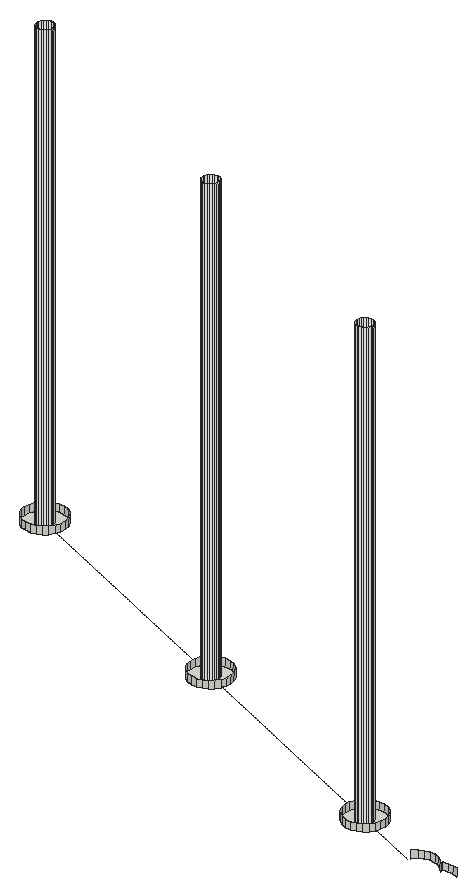
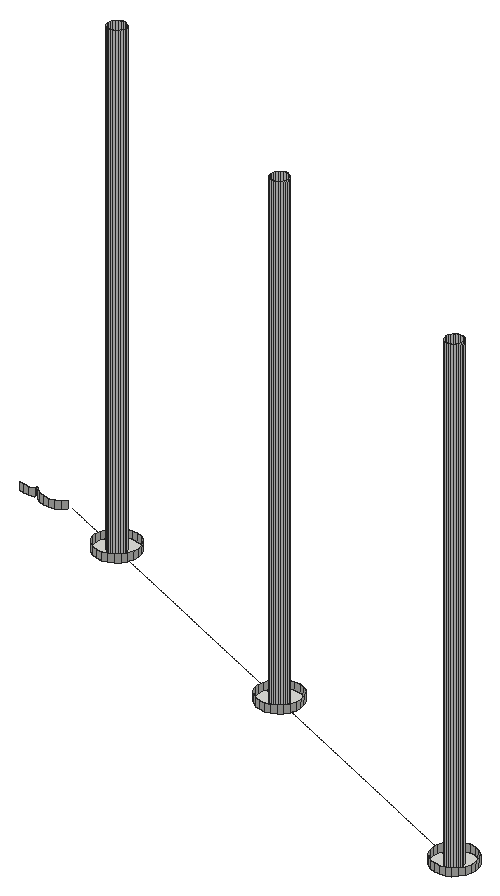
# SketchUp Ruby script. Lengths in inches.
U = 1.inch
M = Sketchup.active_model
def pt(a) = Geom::Point3d.new(a.map { |v| v * U })
def face(e, loops, mat)
  f = e.add_face(loops[0].map { |a| pt(a) })
  loops[1..].each { |l| e.add_face(l.map { |a| pt(a) }).erase! }
  f.material = f.back_material = mat if mat
  f
end
# faces: each face lists its corners as indices into pts; further lists are holes
def faces(e, pts, list, mat = nil) = list.each { |f| face(e, (f[0].is_a?(Array) ? f : [f]).map { |l| l.map { |i| pts[i] } }, mat) }
# xy, xz, yz: faces in a plane at the given z, y or x. An outline is a flat list of corners, or four numbers for a rectangle; further outlines are holes
def ring(l) = l.size == 4 ? [[l[0], l[1]], [l[2], l[1]], [l[2], l[3]], [l[0], l[3]]] : l.each_slice(2).to_a
def flat(e, list, mat, &to3) = list.each { |f| face(e, (f[0].is_a?(Array) ? f : [f]).map { |l| ring(l).map { |u, v| to3.(u, v) } }, mat) }
def xy(e, z, list, mat = nil) = flat(e, list, mat) { |x, y| [x, y, z] }
def xz(e, y, list, mat = nil) = flat(e, list, mat) { |x, z| [x, y, z] }
def yz(e, x, list, mat = nil) = flat(e, list, mat) { |y, z| [x, y, z] }
def lines(e, pts, list) = list.each { |a, b| e.add_line(pt(pts[a]), pt(pts[b])) }
# prism: a flat outline (further loops are holes) pulled along v
def prism(e, loops, v, mat = nil)
  f = face(e, loops, mat); d = Geom::Vector3d.new(v.map { |x| x * U })
  f.pushpull(f.normal.samedirection?(d) ? d.length : -d.length)
end
def box(e, o, s, mat = nil) = prism(e, [[o, [o[0] + s[0], o[1], o[2]], [o[0] + s[0], o[1] + s[1], o[2]], [o[0], o[1] + s[1], o[2]]]], [0, 0, s[2]], mat)
def at(x, y, z, deg = 0) = Geom::Transformation.translation(pt([x, y, z])) * Geom::Transformation.rotation(ORIGIN, Z_AXIS, deg.degrees)
def axes(o, x, y, z) = Geom::Transformation.new([*x, 0, *y, 0, *z, 0, *pt(o).to_a, 1])
def part(name) = M.definitions.add(name)
# library, detail: a bought-in or finely detailed component or shape, given as its bounding box
def library(name, o, s) = part(name).tap { |d| box(d.entities, o, s) }
def detail(e, o, s) = box(e.add_group.entities, o, s)
def put(e, d, t, mat = nil) = e.add_instance(d, t).tap { |i| i.material = mat if mat }
def group(e, t, mat = nil) = e.add_group.tap { |g| g.transformation = t; g.material = mat if mat }.entities
root = M.entities
M.materials.add("[Color_000]").color = [255, 255, 255]
xy(root,321.27,[[1015.61,1014.57,1015.2,1014.59,1014.81,1014.72,1014.46,1014.95,1014.19,1015.26,1014.01,1015.62,1013.92,1016.03,1013.95,1016.4375,1014.06,1016.76,1014.92,1016.39,1014.875,1016.26,1014.87,1016.09,1014.9,1015.93,1014.97,1015.78,1015.08,1015.66,1015.22,1015.57,1015.375,1015.52,1015.54,1015.51,1015.7,1015.54,1015.85,1015.62,1015.97,1015.73,1016.0625,1015.86,1016.07,1015.89,1016.93,1015.51,1016.91,1015.45,1016.6875,1015.11,1016.38,1014.83,1016.01,1014.65],[[1015.61,1014.57,1015.2,1014.59,1014.81,1014.72,1014.46,1014.95,1014.19,1015.26,1014.01,1015.62,1013.92,1016.03,1013.95,1016.4375,1014.06,1016.76,1014.08,1016.83,1014.3,1017.17,1014.61,1017.44,1014.98,1017.625,1015.38,1017.71,1015.79,1017.68,1016.18,1017.55,1016.53,1017.33,1016.8,1017.02,1016.98,1016.65,1017.07,1016.25,1017.04,1015.84,1016.91,1015.45,1016.6875,1015.11,1016.38,1014.83,1016.01,1014.65],[1015.54,1015.51,1015.7,1015.54,1015.85,1015.62,1015.97,1015.73,1016.0625,1015.86,1016.07,1015.89,1016.11,1016.02,1016.125,1016.18,1016.09,1016.34,1016.02,1016.49,1015.91,1016.61,1015.77,1016.7,1015.61,1016.76,1015.45,1016.77,1015.29,1016.73,1015.14,1016.66,1015.02,1016.55,1014.93,1016.41,1014.92,1016.39,1014.875,1016.26,1014.87,1016.09,1014.9,1015.93,1014.97,1015.78,1015.08,1015.66,1015.22,1015.57,1015.375,1015.52]],[996.48,1022.9,996.07,1022.92,995.67,1023.05,995.33,1023.28,995.06,1023.59,994.875,1023.96,994.79,1024.36,994.82,1024.77,994.93,1025.1,995.79,1024.72,995.74,1024.59,995.73,1024.43,995.77,1024.26,995.84,1024.12,995.95,1023.99,996.09,1023.9,996.24,1023.85,996.41,1023.84,996.57,1023.875,996.72,1023.95,996.84,1024.06,996.93,1024.2,996.9375,1024.22,997.8,1023.84,997.78,1023.78,997.55,1023.44,997.25,1023.17,996.88,1022.98],[[996.48,1022.9,996.07,1022.92,995.67,1023.05,995.33,1023.28,995.06,1023.59,994.875,1023.96,994.79,1024.36,994.82,1024.77,994.95,1025.16,995.17,1025.5,995.48,1025.77,995.85,1025.96,996.25,1026.04,996.66,1026.02,997.05,1025.89,997.39,1025.66,997.67,1025.35,997.85,1024.99,997.93,1024.58,997.91,1024.17,997.78,1023.78,997.55,1023.44,997.25,1023.17,996.88,1022.98],[996.41,1023.84,996.57,1023.875,996.72,1023.95,996.84,1024.06,996.93,1024.2,996.9375,1024.22,996.98,1024.35,996.99,1024.52,996.96,1024.68,996.88,1024.82,996.78,1024.95,996.64,1025.04,996.48,1025.09,996.32,1025.1,996.16,1025.07,996.01,1024.99,995.89,1024.88,995.8,1024.75,995.79,1024.72,995.74,1024.59,995.73,1024.43,995.77,1024.26,995.84,1024.12,995.95,1023.99,996.09,1023.9,996.24,1023.85]],[975.89,1031.86,975.48,1031.89,975.09,1032.02,974.75,1032.24,974.48,1032.55,974.29,1032.92,974.21,1033.32,974.23,1033.73,974.34,1034.0625,975.21,1033.69,975.16,1033.55,975.15,1033.39,975.19,1033.23,975.26,1033.08,975.37,1032.96,975.51,1032.87,975.66,1032.82,975.83,1032.81,975.99,1032.84,976.13,1032.91,976.26,1033.02,976.35,1033.16,976.36,1033.18,977.22,1032.81,977.2,1032.75,976.97,1032.4,976.66,1032.13,976.3,1031.95],
  [[975.89,1031.86,975.48,1031.89,975.09,1032.02,974.75,1032.24,974.48,1032.55,974.29,1032.92,974.21,1033.32,974.23,1033.73,974.34,1034.0625,974.36,1034.12,974.59,1034.47,974.9,1034.74,975.27,1034.92,975.67,1035.01,976.08,1034.98,976.47,1034.85,976.8125,1034.625,977.08,1034.32,977.27,1033.95,977.35,1033.55,977.33,1033.14,977.2,1032.75,976.97,1032.4,976.66,1032.13,976.3,1031.95],[975.83,1032.81,975.99,1032.84,976.13,1032.91,976.26,1033.02,976.35,1033.16,976.36,1033.18,976.4,1033.32,976.41,1033.48,976.375,1033.64,976.3,1033.79,976.19,1033.91,976.06,1034,975.9,1034.05,975.74,1034.0625,975.57,1034.03,975.43,1033.96,975.3,1033.85,975.21,1033.71,975.21,1033.69,975.16,1033.55,975.15,1033.39,975.19,1033.23,975.26,1033.08,975.37,1032.96,975.51,1032.87,975.66,1032.82]]])
xy(root,321.27,[[1015.54,1015.51,1015.375,1015.52,1015.22,1015.57,1015.08,1015.66,1014.97,1015.78,1014.9,1015.93,1014.87,1016.09,1014.875,1016.26,1014.92,1016.39,1016.07,1015.89,1016.0625,1015.86,1015.97,1015.73,1015.85,1015.62,1015.7,1015.54],[1016.07,1015.89,1014.92,1016.39,1014.93,1016.41,1015.02,1016.55,1015.14,1016.66,1015.29,1016.73,1015.45,1016.77,1015.61,1016.76,1015.77,1016.7,1015.91,1016.61,1016.02,1016.49,1016.09,1016.34,1016.125,1016.18,1016.11,1016.02],[996.41,1023.84,996.24,1023.85,996.09,1023.9,995.95,1023.99,995.84,1024.12,995.77,1024.26,995.73,1024.43,995.74,1024.59,995.79,1024.72,996.9375,1024.22,996.93,1024.2,996.84,1024.06,996.72,1023.95,996.57,1023.875],[996.9375,1024.22,995.79,1024.72,995.8,1024.75,995.89,1024.88,996.01,1024.99,996.16,1025.07,996.32,1025.1,996.48,1025.09,996.64,1025.04,996.78,1024.95,996.88,1024.82,996.96,1024.68,996.99,1024.52,996.98,1024.35],[975.83,1032.81,975.66,1032.82,975.51,1032.87,975.37,1032.96,975.26,1033.08,975.19,1033.23,975.15,1033.39,975.16,1033.55,975.21,1033.69,976.36,1033.18,976.35,1033.16,976.26,1033.02,976.13,1032.91,975.99,1032.84],
  [976.36,1033.18,975.21,1033.69,975.21,1033.71,975.3,1033.85,975.43,1033.96,975.57,1034.03,975.74,1034.0625,975.9,1034.05,976.06,1034,976.19,1033.91,976.3,1033.79,976.375,1033.64,976.41,1033.48,976.4,1033.32]],"[Color_000]")
p = [[1023.37,1013.92,321.27],[1023.24,1014.07,321.27],[1023.09,1014.23,321.27],[1023.09,1014.23,321.86],[1023.24,1014.07,321.86],[1023.37,1013.92,321.86],
  [1021.18,1014.34,321.27],[1020.87,1014.07,321.27],[1020.87,1014.07,321.86],[1021.18,1014.34,321.86],[1023.77,1014.21,321.27],[1023.36,1014.13,321.27],
  [1023.36,1014.13,321.86],[1023.77,1014.21,321.86],[1024.57,1014.0625,321.27],[1024.18,1014.19,321.27],[1024.18,1014.19,321.86],[1024.57,1014.0625,321.86],
  [1022.75,1014.46,321.27],[1022.75,1014.46,321.86],[1021.55,1014.53,321.27],[1021.55,1014.53,321.86],[1021.95,1014.61,321.27],[1021.95,1014.61,321.86],
  [1022.36,1014.59,321.27],[1022.36,1014.59,321.86],[1014.81,1014.72,321.27],[1015.2,1014.59,321.27],[1015.2,1014.59,321.86],[1014.81,1014.72,321.86],
  [1015.61,1014.57,321.27],[1015.61,1014.57,321.86],[1016.01,1014.65,321.27],[1016.01,1014.65,321.86],[1016.38,1014.83,321.27],[1016.38,1014.83,321.86],
  [1014.46,1014.95,321.27],[1014.46,1014.95,321.86],[1016.6875,1015.11,321.27],[1016.6875,1015.11,321.86],[1014.19,1015.26,321.27],[1014.19,1015.26,321.86],
  [1016.91,1015.45,321.27],[1016.91,1015.45,321.86],[1014.01,1015.62,321.27],[1014.01,1015.62,321.86],[1015.22,1015.57,321.27],[1015.375,1015.52,321.27],
  [1015.375,1015.52,357.27],[1015.22,1015.57,357.27],[1015.54,1015.51,321.27],[1015.54,1015.51,357.27],[1015.7,1015.54,321.27],[1015.7,1015.54,357.27],
  [1015.85,1015.62,321.27],[1015.85,1015.62,357.27],[1016.93,1015.51,321.27],[1017.04,1015.84,321.27],[1017.04,1015.84,321.86],[1013.92,1016.03,321.27],
  [1013.92,1016.03,321.86],[1015.08,1015.66,321.27],[1015.08,1015.66,357.27],[1015.97,1015.73,321.27],[1015.97,1015.73,357.27],[1014.97,1015.78,321.27],
  [1014.97,1015.78,357.27],[1016.0625,1015.86,321.27],[1016.0625,1015.86,357.27],[1014.9,1015.93,321.27],[1014.9,1015.93,357.27],[1017.07,1016.25,321.27],
  [1017.07,1016.25,321.86],[1014.87,1016.09,321.27],[1014.87,1016.09,357.27],[1016.07,1015.89,321.27],[1016.11,1016.02,321.27],[1016.11,1016.02,357.27],
  [1013.95,1016.4375,321.27],[1013.95,1016.4375,321.86],[1016.125,1016.18,321.27],[1016.125,1016.18,357.27],[1014.875,1016.26,321.27],[1014.875,1016.26,357.27],
  [1016.09,1016.34,321.27],[1016.09,1016.34,357.27],[1014.93,1016.41,321.27],[1014.92,1016.39,321.27],[1014.93,1016.41,357.27],[1016.02,1016.49,321.27],
  [1016.02,1016.49,357.27],[1016.98,1016.65,321.27],[1016.98,1016.65,321.86],[1014.08,1016.83,321.27],[1014.06,1016.76,321.27],[1014.08,1016.83,321.86],
  [1015.02,1016.55,321.27],[1015.02,1016.55,357.27],[1015.91,1016.61,321.27],[1015.91,1016.61,357.27],[1015.14,1016.66,321.27],[1015.14,1016.66,357.27],
  [1015.77,1016.7,321.27],[1015.77,1016.7,357.27],[1015.29,1016.73,321.27],[1015.29,1016.73,357.27],[1015.45,1016.77,321.27],[1015.45,1016.77,357.27],
  [1015.61,1016.76,321.27],[1015.61,1016.76,357.27],[1016.8,1017.02,321.27],[1016.8,1017.02,321.86],[1014.3,1017.17,321.27],[1014.3,1017.17,321.86],
  [1016.53,1017.33,321.27],[1016.53,1017.33,321.86],[1014.61,1017.44,321.27],[1014.61,1017.44,321.86],[1016.18,1017.55,321.27],[1016.18,1017.55,321.86],
  [1014.98,1017.625,321.27],[1014.98,1017.625,321.86],[1015.38,1017.71,321.27],[1015.38,1017.71,321.86],[1015.79,1017.68,321.27],[1015.79,1017.68,321.86],
  [995.67,1023.05,321.27],[996.07,1022.92,321.27],[996.07,1022.92,321.86],[995.67,1023.05,321.86],[996.48,1022.9,321.27],[996.48,1022.9,321.86],
  [996.88,1022.98,321.27],[996.88,1022.98,321.86],[997.25,1023.17,321.27],[997.25,1023.17,321.86],[995.33,1023.28,321.27],[995.33,1023.28,321.86],
  [997.55,1023.44,321.27],[997.55,1023.44,321.86],[995.06,1023.59,321.27],[995.06,1023.59,321.86],[997.78,1023.78,321.27],[997.78,1023.78,321.86],
  [994.875,1023.96,321.27],[994.875,1023.96,321.86],[996.24,1023.85,321.27],[996.41,1023.84,321.27],[996.41,1023.84,357.27],[996.24,1023.85,357.27],
  [996.57,1023.875,321.27],[996.57,1023.875,357.27],[997.8,1023.84,321.27],[997.91,1024.17,321.27],[997.91,1024.17,321.86],[995.95,1023.99,321.27],
  [996.09,1023.9,321.27],[996.09,1023.9,357.27],[995.95,1023.99,357.27],[996.72,1023.95,321.27],[996.72,1023.95,357.27],[996.84,1024.06,321.27],
  [996.84,1024.06,357.27],[994.79,1024.36,321.27],[994.79,1024.36,321.86],[995.84,1024.12,321.27],[995.84,1024.12,357.27],[995.77,1024.26,321.27],
  [995.77,1024.26,357.27],[996.93,1024.2,321.27],[996.93,1024.2,357.27],[996.9375,1024.22,321.27],[996.98,1024.35,321.27],[996.98,1024.35,357.27],
  [997.93,1024.58,321.27],[997.93,1024.58,321.86],[995.73,1024.43,321.27],[995.73,1024.43,357.27],[994.82,1024.77,321.27],[994.82,1024.77,321.86],
  [995.74,1024.59,321.27],[995.74,1024.59,357.27],[996.99,1024.52,321.27],[996.99,1024.52,357.27],[996.96,1024.68,321.27],[996.96,1024.68,357.27],
  [995.8,1024.75,321.27],[995.79,1024.72,321.27],[995.8,1024.75,357.27],[997.85,1024.99,321.27],[997.85,1024.99,321.86],[995.89,1024.88,321.27],
  [995.89,1024.88,357.27],[996.88,1024.82,321.27],[996.88,1024.82,357.27],[994.95,1025.16,321.27],[994.93,1025.1,321.27],[994.95,1025.16,321.86],
  [996.78,1024.95,321.27],[996.78,1024.95,357.27],[996.01,1024.99,321.27],[996.01,1024.99,357.27],[996.64,1025.04,321.27],[996.64,1025.04,357.27],
  [996.16,1025.07,321.27],[996.16,1025.07,357.27],[996.48,1025.09,321.27],[996.48,1025.09,357.27],[997.67,1025.35,321.27],[997.67,1025.35,321.86],
  [996.32,1025.1,321.27],[996.32,1025.1,357.27],[995.17,1025.5,321.27],[995.17,1025.5,321.86],[997.39,1025.66,321.27],[997.39,1025.66,321.86],
  [995.48,1025.77,321.27],[995.48,1025.77,321.86],[997.05,1025.89,321.27],[997.05,1025.89,321.86],[995.85,1025.96,321.27],[995.85,1025.96,321.86],
  [996.66,1026.02,321.27],[996.66,1026.02,321.86],[996.25,1026.04,321.27],[996.25,1026.04,321.86],[975.09,1032.02,321.27],[975.48,1031.89,321.27],
  [975.48,1031.89,321.86],[975.09,1032.02,321.86],[975.89,1031.86,321.27],[975.89,1031.86,321.86],[976.3,1031.95,321.27],[976.3,1031.95,321.86],
  [976.66,1032.13,321.27],[976.66,1032.13,321.86],[974.75,1032.24,321.27],[974.75,1032.24,321.86],[976.97,1032.4,321.27],[976.97,1032.4,321.86],
  [974.48,1032.55,321.27],[974.48,1032.55,321.86],[977.2,1032.75,321.27],[977.2,1032.75,321.86],[974.29,1032.92,321.27],[974.29,1032.92,321.86],
  [977.22,1032.81,321.27],[977.33,1033.14,321.27],[977.33,1033.14,321.86],[975.51,1032.87,321.27],[975.66,1032.82,321.27],[975.66,1032.82,357.27],
  [975.51,1032.87,357.27],[975.83,1032.81,321.27],[975.83,1032.81,357.27],[975.99,1032.84,321.27],[975.99,1032.84,357.27],[976.13,1032.91,321.27],
  [976.13,1032.91,357.27],[974.21,1033.32,321.27],[974.21,1033.32,321.86],[975.37,1032.96,321.27],[975.37,1032.96,357.27],[976.26,1033.02,321.27],
  [976.26,1033.02,357.27],[975.26,1033.08,321.27],[975.26,1033.08,357.27],[976.35,1033.16,321.27],[976.35,1033.16,357.27],[975.19,1033.23,321.27],
  [975.19,1033.23,357.27],[977.35,1033.55,321.27],[977.35,1033.55,321.86],[975.15,1033.39,321.27],[975.15,1033.39,357.27],[976.36,1033.18,321.27],
  [976.4,1033.32,321.27],[976.4,1033.32,357.27],[974.23,1033.73,321.27],[974.23,1033.73,321.86],[976.41,1033.48,321.27],[976.41,1033.48,357.27],
  [975.16,1033.55,321.27],[975.16,1033.55,357.27],[976.375,1033.64,321.27],[976.375,1033.64,357.27],[977.27,1033.95,321.27],[977.27,1033.95,321.86],
  [975.21,1033.71,321.27],[975.21,1033.69,321.27],[975.21,1033.71,357.27],[976.3,1033.79,321.27],[976.3,1033.79,357.27],[974.36,1034.12,321.27],
  [974.34,1034.0625,321.27],[974.36,1034.12,321.86],[975.3,1033.85,321.27],[975.3,1033.85,357.27],[975.43,1033.96,321.27],[975.43,1033.96,357.27],
  [976.19,1033.91,321.27],[976.19,1033.91,357.27],[976.06,1034,321.27],[976.06,1034,357.27],[975.57,1034.03,321.27],[975.57,1034.03,357.27],
  [975.74,1034.0625,321.27],[975.74,1034.0625,357.27],[975.9,1034.05,321.27],[975.9,1034.05,357.27],[977.08,1034.32,321.27],[977.08,1034.32,321.86],
  [974.59,1034.47,321.27],[974.59,1034.47,321.86],[976.8125,1034.625,321.27],[976.8125,1034.625,321.86],[974.9,1034.74,321.27],[974.9,1034.74,321.86],
  [976.47,1034.85,321.27],[976.47,1034.85,321.86],[975.27,1034.92,321.27],[975.27,1034.92,321.86],[975.67,1035.01,321.27],[975.67,1035.01,321.86],
  [976.08,1034.98,321.27],[976.08,1034.98,321.86],[1020.73,1013.86,321.27]]
faces(root,p,[[0,1,2,3,4,5],[6,7,8,9],[10,11,12,13],[14,15,16,17],[2,18,19,3],[15,10,13,16],[20,6,9,21],[22,20,21,23],
  [18,24,25,19],[26,27,28,29],[27,30,31,28],[30,32,33,31],[32,34,35,33],[24,22,23,25],[36,26,29,37],[34,38,39,35],
  [40,36,37,41],[38,42,43,39],[44,40,41,45],[42,56,57,58,43],[59,44,45,60],[57,71,72,58],[78,59,60,79],[71,91,92,72],
  [93,94,78,79,95],[91,110,111,92],[112,93,95,113],[110,114,115,111],[116,112,113,117],[114,118,119,115],[120,116,117,121],[122,120,121,123],
  [118,124,125,119],[124,122,123,125],[126,127,128,129],[127,130,131,128],[130,132,133,131],[132,134,135,133],[136,126,129,137],[134,138,139,135],
  [140,136,137,141],[138,142,143,139],[144,140,141,145],[142,152,153,154,143],[163,144,145,164],[153,174,175,154],[178,163,164,179],[174,189,190,175],
  [195,196,178,179,197],[189,208,209,190],[212,195,197,213],[208,214,215,209],[216,212,213,217],[214,218,219,215],[220,216,217,221],[218,222,223,219],
  [224,220,221,225],[222,224,225,223],[226,227,228,229],[227,230,231,228],[230,232,233,231],[232,234,235,233],[236,226,229,237],[234,238,239,235],
  [240,236,237,241],[238,242,243,239],[244,240,241,245],[242,246,247,248,243],[259,244,245,260],[247,271,272,248],[278,259,260,279],[271,286,287,272],
  [293,294,278,279,295],[286,310,311,287],[312,293,295,313],[310,314,315,311],[316,312,313,317],[314,318,319,315],[320,316,317,321],[322,320,321,323],
  [318,324,325,319],[324,322,323,325]])
faces(root,p,[[46,47,48,49],[47,50,51,48],[50,52,53,51],[52,54,55,53],[61,46,49,62],[54,63,64,55],[65,61,62,66],[63,67,68,64],
  [69,65,66,70],[73,69,70,74],[67,75,76,77,68],[76,80,81,77],[82,73,74,83],[80,84,85,81],[86,87,82,83,88],[84,89,90,85],
  [96,86,88,97],[89,98,99,90],[100,96,97,101],[98,102,103,99],[104,100,101,105],[106,104,105,107],[102,108,109,103],[108,106,107,109],
  [146,147,148,149],[147,150,151,148],[155,156,157,158],[156,146,149,157],[150,159,160,151],[159,161,162,160],[165,155,158,166],[167,165,166,168],
  [161,169,170,162],[169,171,172,173,170],[176,167,168,177],[180,176,177,181],[172,182,183,173],[182,184,185,183],[186,187,180,181,188],[191,186,188,192],
  [184,193,194,185],[193,198,199,194],[200,191,192,201],[198,202,203,199],[204,200,201,205],[202,206,207,203],[210,204,205,211],[206,210,211,207],
  [249,250,251,252],[250,253,254,251],[253,255,256,254],[255,257,258,256],[261,249,252,262],[257,263,264,258],[265,261,262,266],[263,267,268,264],
  [269,265,266,270],[273,269,270,274],[267,275,276,277,268],[276,280,281,277],[282,273,274,283],[280,284,285,281],[288,289,282,283,290],[284,291,292,285],
  [296,288,290,297],[298,296,297,299],[291,300,301,292],[300,302,303,301],[304,298,299,305],[306,304,305,307],[302,308,309,303],[308,306,307,309]],"[Color_000]")
lines(root,p,[[196,246],[94,152],[326,56]])
